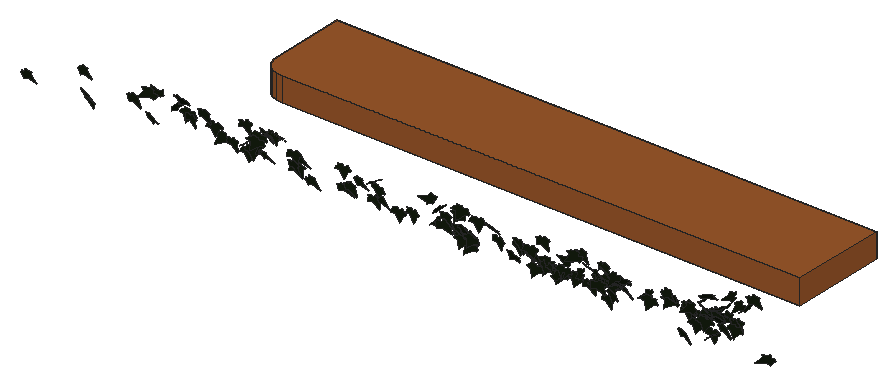
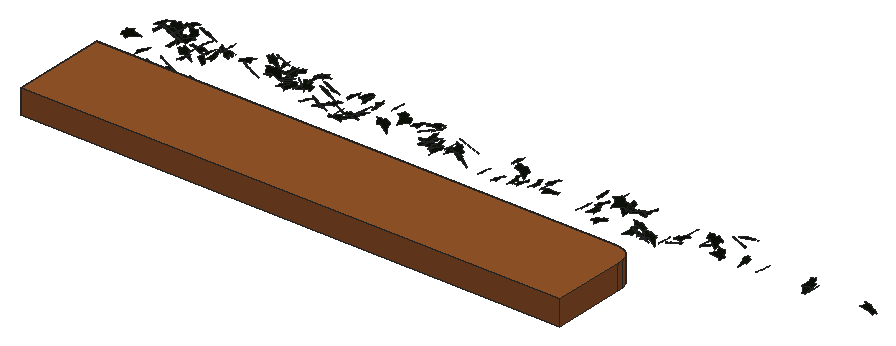
# SketchUp Ruby script. Lengths in millimetres.
U = 1.mm
M = Sketchup.active_model
def pt(a) = Geom::Point3d.new(a.map { |v| v * U })
def face(e, loops, mat)
  f = e.add_face(loops[0].map { |a| pt(a) })
  loops[1..].each { |l| e.add_face(l.map { |a| pt(a) }).erase! }
  f.material = f.back_material = mat if mat
  f
end
# faces: each face lists its corners as indices into pts; further lists are holes
def faces(e, pts, list, mat = nil) = list.each { |f| face(e, (f[0].is_a?(Array) ? f : [f]).map { |l| l.map { |i| pts[i] } }, mat) }
# xy, xz, yz: faces in a plane at the given z, y or x. An outline is a flat list of corners, or four numbers for a rectangle; further outlines are holes
def ring(l) = l.size == 4 ? [[l[0], l[1]], [l[2], l[1]], [l[2], l[3]], [l[0], l[3]]] : l.each_slice(2).to_a
def flat(e, list, mat, &to3) = list.each { |f| face(e, (f[0].is_a?(Array) ? f : [f]).map { |l| ring(l).map { |u, v| to3.(u, v) } }, mat) }
def xy(e, z, list, mat = nil) = flat(e, list, mat) { |x, y| [x, y, z] }
def xz(e, y, list, mat = nil) = flat(e, list, mat) { |x, z| [x, y, z] }
def yz(e, x, list, mat = nil) = flat(e, list, mat) { |y, z| [x, y, z] }
def lines(e, pts, list) = list.each { |a, b| e.add_line(pt(pts[a]), pt(pts[b])) }
# prism: a flat outline (further loops are holes) pulled along v
def prism(e, loops, v, mat = nil)
  f = face(e, loops, mat); d = Geom::Vector3d.new(v.map { |x| x * U })
  f.pushpull(f.normal.samedirection?(d) ? d.length : -d.length)
end
def box(e, o, s, mat = nil) = prism(e, [[o, [o[0] + s[0], o[1], o[2]], [o[0] + s[0], o[1] + s[1], o[2]], [o[0], o[1] + s[1], o[2]]]], [0, 0, s[2]], mat)
def at(x, y, z, deg = 0) = Geom::Transformation.translation(pt([x, y, z])) * Geom::Transformation.rotation(ORIGIN, Z_AXIS, deg.degrees)
def axes(o, x, y, z) = Geom::Transformation.new([*x, 0, *y, 0, *z, 0, *pt(o).to_a, 1])
def part(name) = M.definitions.add(name)
# library, detail: a bought-in or finely detailed component or shape, given as its bounding box
def library(name, o, s) = part(name).tap { |d| box(d.entities, o, s) }
def detail(e, o, s) = box(e.add_group.entities, o, s)
def put(e, d, t, mat = nil) = e.add_instance(d, t).tap { |i| i.material = mat if mat }
def group(e, t, mat = nil) = e.add_group.tap { |g| g.transformation = t; g.material = mat if mat }.entities
root = M.entities
M.materials.add("Emissive").color = [255, 185, 108]
M.materials.add("[Wood Cherry Original]").color = [152, 86, 42]
M.materials.add("efeu1").color = [18, 25, 13]
c1 = part("ivyleaf_9")
p = [[39.1,54.8,31.7],[34.5,51.8,30.2],[-5.3,25.2,17.3],[-17.9,28.3,20.9],[-21.6,21.7,17],[-20.2,4.3,5.3],
  [-22.9,-0.3,2.5],[-17.1,-4,-0.6],[-2,-2.1,-1.2],[-0.7,-15.4,-10.1],[16.6,-22.3,-16.7],[21.1,-15.1,-12.5],
  [32.7,-10.7,-11],[46.1,-1.8,-6.6],[30.8,11.2,3.8]]
faces(c1.entities,p,[[0,1,2,3,4,5,6,7,8,9,10,11,12,13,14]],"efeu1")
put(root,c1,axes([8074.5,526.7,5825.1],[-2.17662,-0.89017,-0.15094],[0.20307,0.10863,-1.44912],[1.70631,-1.14845,-0.02008]))
put(root,c1,axes([2613.1,371,5827.4],[0.23892,-1.21301,0.85578],[0.50011,-0.82712,-1.21092],[2.78069,0.25298,0.14425]))
put(root,c1,axes([6163.8,513.2,5830],[-0.62934,-1.41671,-0.06953],[0.03051,0.06765,-1.45479],[2.69936,-0.33106,0.00023]))
put(root,c1,axes([4921.2,550.8,5850.1],[-0.48361,-1.23805,-0.68713],[0.5351,0.64009,-1.25727],[2.64118,-0.35637,0.12891]))
put(root,c1,axes([10571.6,482.2,5821.8],[-0.21337,-0.04901,-1.49779],[-0.24319,-1.49619,0.05852],[-2.84173,0.13172,0.10745]))
put(root,c1,axes([5168,430.4,5854.4],[1.26122,-1.15667,-0.60639],[-0.06808,0.66366,-1.305],[2.48461,0.60532,0.27205]))
put(root,c1,axes([7115.8,397.2,5845.3],[-2.66405,-0.3276,-0.31618],[0.57453,0.09743,-1.43737],[0.64867,-1.43173,-0.02547]))
put(root,c1,axes([9847.7,543.6,5834.5],[-0.34368,-1.44406,-0.07033],[0.01652,0.06979,-1.45531],[2.75154,-0.18079,-0.00005]))
put(root,c1,axes([9623.6,355.2,5836.9],[1.52236,-1.2895,-0.02319],[-0.02465,0.01926,-1.51744],[2.45444,0.8,-0.00086]))
put(root,c1,axes([9922.6,457.9,5853.9],[-0.55823,1.32512,-0.53209],[0.00313,-0.54288,-1.35291],[-2.71768,-0.27281,0.10774]))
put(root,c1,axes([4382.2,525,5839.3],[-0.82714,-1.39965,0.00399],[0.04642,-0.01175,-1.46533],[2.66342,-0.43447,0.02677]))
put(root,c1,axes([6959.6,472.3,5852.5],[-1.32426,-1.09577,0.67655],[-0.32073,-0.6849,-1.28261],[2.42986,-0.68759,0.19942]))
put(root,c1,axes([4525.8,533.9,5858.8],[1.99885,-0.95702,-0.27557],[0.05319,0.42865,-1.38215],[1.89465,0.99761,0.32952]))
put(root,c1,axes([8422.7,503.1,5866.6],[-0.20032,-1.44792,-0.35467],[0.41494,0.33678,-1.43958],[2.80664,-0.15313,0.18752]))
put(root,c1,axes([7991.5,519.2,5862.7],[-0.53308,-1.41745,0.3331],[0.07754,-0.3467,-1.44108],[2.77009,-0.26307,0.10444]))
put(root,c1,axes([7929.3,514.9,5863.4],[-1.43561,-1.20456,0.40338],[-0.27216,-0.38564,-1.41898],[2.40228,-0.76354,0.0803]))
put(root,c1,axes([6307.3,534.6,5861.2],[-0.30689,-1.42825,0.19482],[-0.00237,-0.1959,-1.43718],[2.74342,-0.15994,0.02055]))
put(root,c1,axes([4417,538.3,5860.9],[-0.70879,-1.41411,0.01021],[0.03058,-0.01479,-1.4622],[2.69123,-0.37227,0.0193]))
put(root,c1,axes([5883.1,495.2,5879.9],[-0.07528,-1.37857,-0.49737],[0.17964,0.49412,-1.37707],[2.78344,-0.06918,0.07542]))
put(root,c1,axes([6883.1,502.8,5885.4],[0.2677,-1.15782,-0.88511],[-0.14456,0.88219,-1.16607],[2.76992,0.15794,0.02468]))
put(root,c1,axes([8271.9,523.6,5867.7],[-1.60859,-1.20404,0.15445],[0.05883,-0.20949,-1.46393],[2.30957,-0.83327,0.14486]))
put(root,c1,axes([8722,394,5865.9],[0.2362,-1.49888,0.06118],[0.01867,-0.06058,-1.504],[2.85498,0.1244,0.00477]))
put(root,c1,axes([7871.1,416.1,5870.6],[-1.47445,-1.21466,0.2883],[-0.02362,-0.33179,-1.43125],[2.37585,-0.75712,0.16469]))
put(root,c1,axes([7021.3,395.5,5873.9],[-1.28203,-1.19407,0.51458],[-0.15548,-0.53952,-1.35889],[2.4697,-0.65381,0.18157]))
put(root,c1,axes([9462.2,931.6,5866.9],[-0.51812,1.43082,-0.02284],[0.00789,-0.02246,-1.45649],[-2.72347,-0.27227,0.00013]))
put(root,c1,axes([8039.8,520.9,5871.8],[0.22661,-1.47073,0.13778],[-0.05792,-0.14064,-1.47496],[2.81075,0.11568,-0.0415]))
put(root,c1,axes([4099.7,526.8,5877.1],[-2.19562,-0.7999,0.43441],[-0.20382,-0.57717,-1.34716],[1.72035,-1.08926,0.39482]))
put(root,c1,axes([4496.7,550.6,5873.1],[-1.75881,1.11126,0.13863],[-0.41166,-0.00076,-1.43574],[-2.09121,-0.93447,0.16603]))
put(root,c1,axes([7050.9,474.1,5872.4],[-1.72475,-1.171,0.03617],[-0.0141,-0.04,-1.48059],[2.22966,-0.90608,0.01862]))
put(root,c1,axes([4176.2,525.2,5876.1],[0.50051,-1.4373,-0.12505],[-0.02862,0.12437,-1.46114],[2.74565,0.26331,0.00756]))
put(root,c1,axes([5544.9,482,5895.5],[-0.4571,-0.98003,-1.02974],[1.52498,0.7693,-0.91904],[2.23476,-0.72541,0.41653]))
put(root,c1,axes([9716.5,887,5870.4],[0.60839,0.8956,1.13524],[0.51702,1.10475,-0.94804],[-2.703,0.4129,0.07418]))
put(root,c1,axes([8131,418.2,5854.4],[-2.2074,0.66073,-0.71144],[-1.17316,0.35523,1.33483],[1.4277,1.31346,-0.00312]))
put(root,c1,axes([3324.1,363,5901.2],[2.09552,-0.55116,-0.78981],[-0.96665,0.68695,-1.18744],[1.55738,1.16799,0.32569]))
put(root,c1,axes([7589,423,5899.1],[1.51499,0.20162,-1.26609],[-2.40335,-0.13395,-0.81528],[-0.42119,1.48953,0.09806]))
put(root,c1,axes([1891.2,333.9,5872.9],[-0.0723,-0.29316,-1.43905],[2.73532,0.2886,-0.09674],[0.57478,-1.41032,0.27934]))
put(root,c1,axes([5937.2,506.4,5895.8],[1.53147,-1.19179,-0.37751],[-0.30259,0.34775,-1.43672],[2.35996,0.81799,0.06077]))
put(root,c1,axes([9436.4,936.6,5886.9],[2.0993,0.70408,0.61716],[0.93658,0.37536,-1.30776],[-1.51595,1.20693,0.04669]))
put(root,c1,axes([6643,495.3,5899.6],[-1.47757,1.20987,-0.23901],[0.26921,-0.1932,-1.43746],[-2.33163,-0.78901,-0.01451]))
put(root,c1,axes([4335.5,547.4,5894],[-0.22042,1.44759,-0.09005],[0.03728,-0.08877,-1.45216],[-2.76013,-0.1168,-0.01242]))
put(root,c1,axes([6715,460.8,5920.9],[-0.17939,-1.02389,-1.07244],[0.6259,1.0334,-1.01552],[2.75163,-0.30181,0.16108]))
put(root,c1,axes([9849.8,968.4,5918.2],[-2.41772,0.37642,-0.5762],[0.89977,-0.4018,-1.30481],[-0.95196,-1.33579,0.23011]))
put(root,c1,axes([7923.5,526.7,5903.8],[-2.61277,-0.5316,0.11045],[-0.14737,-0.10556,-1.47049],[1.02279,-1.37322,0.07028]))
put(root,c1,axes([6997.7,484.7,5907.7],[-0.22258,-1.44613,0.25942],[-0.06853,-0.25734,-1.45078],[2.79538,-0.12146,-0.01491]))
put(root,c1,axes([8317.5,520.1,5912],[-2.17254,0.93752,-0.15008],[0.11638,-0.16161,-1.47468],[-1.80326,-1.13994,0.08563]))
put(root,c1,axes([9614,550.8,5895.2],[0.22234,-0.05899,-1.44158],[2.60088,-0.45931,0.12954],[-0.88062,-1.37144,0.01862]))
put(root,c1,axes([2565.1,339.6,5909.3],[2.04119,-1.04548,-0.03075],[-0.04549,0.01953,-1.49776],[1.9901,1.07276,-0.0027]))
put(root,c1,axes([9941.5,963.7,5926.8],[-1.51695,1.11002,-0.49201],[0.38174,-0.46009,-1.36294],[-2.27907,-0.8159,0.09919]))
put(root,c1,axes([5608,472.8,5925.1],[0.49792,-1.37055,-0.38286],[0.00397,0.38965,-1.39341],[2.70829,0.2514,0.07243]))
put(root,c1,axes([9754,454.5,5932.1],[-2.22925,-0.62663,-0.58884],[1.05467,0.21076,-1.3266],[1.25137,-1.29395,0.06909]))
put(root,c1,axes([6870.3,477.7,5919.7],[1.11639,-1.39175,0.06191],[0.04657,-0.05687,-1.51032],[2.651,0.5871,0.00046]))
put(root,c1,axes([8144.7,482.1,5920.5],[-1.36467,-1.27837,0.00389],[0.05068,-0.01939,-1.46537],[2.43248,-0.71679,0.03271]))
put(root,c1,axes([7141.3,383.9,5930.5],[-1.51061,-1.13052,0.5055],[-0.15923,-0.55009,-1.36162],[2.35151,-0.76349,0.23253]))
put(root,c1,axes([9970.5,528,5930.8],[1.20104,-1.31121,-0.15388],[-0.06338,0.15469,-1.4547],[2.51182,0.63086,0.03687]))
put(root,c1,axes([4482.1,512.6,5935.1],[-0.34853,1.39929,0.38168],[-0.66756,0.33057,-1.38019],[-2.67849,-0.26446,0.29432]))
put(root,c1,axes([4942.1,551.1,5945.4],[1.7208,-1.0969,-0.2869],[0.0833,0.40045,-1.3931],[2.15625,0.85992,0.28278]))
put(root,c1,axes([8696.9,515.1,5934.2],[-1.0833,-1.36042,-0.02757],[0.02667,0.02402,-1.47469],[2.58954,-0.56936,0.00365]))
put(root,c1,axes([8563.2,481.2,5935.3],[-1.43694,-0.51266,1.16043],[-1.16352,-1.03622,-0.85555],[2.11562,-0.91809,0.31765]))
put(root,c1,axes([3031.6,481.9,5958.3],[0.83833,-1.33393,-0.39082],[0.08307,0.42305,-1.39473],[2.64416,0.40963,0.16773]))
put(root,c1,axes([6954.7,446.8,5956.1],[1.72062,-1.16045,-0.26707],[-0.15522,0.27419,-1.46747],[2.26098,0.90194,0.1025]))
put(root,c1,axes([5649,542.7,5969.1],[1.50154,-1.17861,-0.33272],[0.008,0.39839,-1.40126],[2.33078,0.75792,0.21916]))
put(root,c1,axes([8629.5,473.5,5969.5],[2.63079,0.44114,-0.2309],[-0.38678,-0.12215,-1.44998],[-0.86511,1.39612,-0.0539]))
put(root,c1,axes([3982,515.9,5974.4],[-0.98985,-1.35354,-0.31276],[0.14012,0.30663,-1.44946],[2.64021,-0.52373,-0.04033]))
put(root,c1,axes([7746.8,467.5,5982.5],[0.91678,-1.36019,-0.41762],[0.15716,0.46688,-1.4254],[2.70341,0.43413,0.22449]))
put(root,c1,axes([9712,547.4,5963.8],[0.16735,-1.44975,0.03493],[0.00077,-0.03497,-1.45241],[2.75996,0.08791,-0.00171]))
put(root,c1,axes([8856.6,311.8,5973.8],[-0.31839,-1.1428,0.94464],[-0.08234,-0.94647,-1.15267],[2.82063,-0.15663,0.07298]))
put(root,c1,axes([6708,513.1,5976.4],[0.53261,-1.4357,-0.1573],[0.07996,0.16825,-1.4609],[2.74762,0.27341,0.07301]))
put(root,c1,axes([2392.4,546.3,5997],[1.0312,-1.18623,-0.64307],[-0.23783,0.64589,-1.29672],[2.55701,0.53846,0.13873]))
put(root,c1,axes([9562,528.4,5979.1],[-0.22617,-1.46967,-0.03001],[-0.08508,0.03371,-1.4737],[2.79636,-0.11784,-0.04726]))
put(root,c1,axes([9130.9,512.3,5978.2],[-2.13533,0.97288,0.0186],[-0.02858,0.01107,-1.48503],[-1.85171,-1.12207,0.00147]))
put(root,c1,axes([8682.7,509.2,5987.9],[-1.85652,-1.0603,0.3972],[0.0186,-0.53214,-1.39653],[2.15483,-0.90892,0.35426]))
put(root,c1,axes([3722.3,483.8,5983.3],[0.46935,-1.45658,0.09217],[0.00557,-0.09299,-1.47725],[2.7777,0.2463,-0.01261]))
put(root,c1,axes([8847.7,461.3,5986.2],[1.66454,-1.19951,0.10159],[0.10933,-0.08385,-1.48451],[2.28848,0.87648,-0.00298]))
put(root,c1,axes([8502.3,495.6,6002.1],[-1.21259,0.12987,-1.35187],[2.24754,-0.68446,-0.62232],[-1.27647,-1.32854,0.18847]))
put(root,c1,axes([9204.3,437.1,5988.4],[-1.61526,-1.22771,0.1124],[-0.1003,-0.1002,-1.49245],[2.34421,-0.85023,0.01359]))
g1 = group(root,at(3881.8,1531.6,5905.3),"[Wood Cherry Original]")
xy(g1,0,[[[6377.5,-209.6,265.9,-209.5,184.6,-202.2,118.2,-180,66.5,-143.1,29.5,-91.4,7.4,-24.9,0,56.3,0,914.4,6377.5,914.4],[4138.7,109.7,4197.4,117.4,4252.2,140.1,4299.2,176.2,4335.3,223.2,4357.9,278,4365.7,336.7,4357.9,395.5,4335.3,450.2,4299.2,497.2,4252.2,533.3,4197.4,556,4138.7,563.7,4079.9,556,4025.1,533.3,3978.1,497.2,3942.1,450.2,3919.4,395.5,3911.6,336.7,3919.4,278,3942.1,223.2,3978.1,176.2,4025.1,140.1,4079.9,117.4],[2346.9,109.7,2405.7,117.4,2460.4,140.1,2507.4,176.2,2543.5,223.2,2566.2,278,2573.9,336.7,2566.2,395.5,2543.5,450.2,2507.4,497.2,2460.4,533.3,2405.7,556,2346.9,563.7,2288.1,556,2233.4,533.3,2186.4,497.2,2150.3,450.2,2127.6,395.5,2119.9,336.7,2127.6,278,2150.3,223.2,2186.4,176.2,2233.4,140.1,2288.1,117.4],[555.1,109.7,613.9,117.4,668.6,140.1,715.7,176.2,751.7,223.2,774.4,278,782.1,336.7,774.4,395.5,751.7,450.2,715.7,497.2,668.6,533.3,613.9,556,555.1,563.7,496.4,556,441.6,533.3,394.6,497.2,358.5,450.2,335.9,395.5,328.1,336.7,335.9,278,358.5,223.2,394.6,176.2,441.6,140.1,496.4,117.4],[5930.4,109.7,5989.2,117.4,6043.9,140.1,6090.9,176.2,6127,223.2,6149.7,278,6157.4,336.7,6149.7,395.5,6127,450.2,6090.9,497.2,6043.9,533.3,5989.2,556,5930.4,563.7,5871.7,556,5816.9,533.3,5769.9,497.2,5733.8,450.2,5711.1,395.5,5703.4,336.7,5711.1,278,5733.8,223.2,5769.9,176.2,5816.9,140.1,5871.7,117.4]],[[555.1,109.7,496.4,117.4,441.6,140.1,394.6,176.2,358.5,223.2,335.9,278,328.1,336.7,335.9,395.5,358.5,450.2,394.6,497.2,441.6,533.3,496.4,556,555.1,563.7,613.9,556,668.6,533.3,715.7,497.2,751.7,450.2,774.4,395.5,782.1,336.7,774.4,278,751.7,223.2,715.7,176.2,668.6,140.1,613.9,117.4],[555.1,166.8,599.1,172.6,640.1,189.6,675.2,216.6,702.2,251.8,719.2,292.7,725,336.7,719.2,380.7,702.2,421.6,675.2,456.8,640.1,483.8,599.1,500.8,555.1,506.6,511.2,500.8,470.2,483.8,435,456.8,408,421.6,391.1,380.7,385.3,336.7,391.1,292.7,408,251.8,435,216.6,470.2,189.6,511.2,172.6]],[[2346.9,109.7,2288.1,117.4,2233.4,140.1,2186.4,176.2,2150.3,223.2,2127.6,278,2119.9,336.7,2127.6,395.5,2150.3,450.2,2186.4,497.2,2233.4,533.3,2288.1,556,2346.9,563.7,2405.7,556,2460.4,533.3,2507.4,497.2,2543.5,450.2,2566.2,395.5,2573.9,336.7,2566.2,278,2543.5,223.2,2507.4,176.2,2460.4,140.1,2405.7,117.4],[2346.9,166.8,2390.9,172.6,2431.8,189.6,2467,216.6,2494,251.8,2511,292.7,2516.8,336.7,2511,380.7,2494,421.6,2467,456.8,2431.8,483.8,2390.9,500.8,2346.9,506.6,2302.9,500.8,2262,483.8,2226.8,456.8,2199.8,421.6,2182.8,380.7,2177,336.7,2182.8,292.7,2199.8,251.8,2226.8,216.6,2262,189.6,2302.9,172.6]],[[4138.7,109.7,4079.9,117.4,4025.1,140.1,3978.1,176.2,3942.1,223.2,3919.4,278,3911.6,336.7,3919.4,395.5,3942.1,450.2,3978.1,497.2,4025.1,533.3,4079.9,556,4138.7,563.7,4197.4,556,4252.2,533.3,4299.2,497.2,4335.3,450.2,4357.9,395.5,4365.7,336.7,4357.9,278,4335.3,223.2,4299.2,176.2,4252.2,140.1,4197.4,117.4],[4138.7,166.8,4182.6,172.6,4223.6,189.6,4258.8,216.6,4285.8,251.8,4302.7,292.7,4308.5,336.7,4302.7,380.7,4285.8,421.6,4258.8,456.8,4223.6,483.8,4182.6,500.8,4138.7,506.6,4094.7,500.8,4053.7,483.8,4018.5,456.8,3991.5,421.6,3974.6,380.7,3968.8,336.7,3974.6,292.7,3991.5,251.8,4018.5,216.6,4053.7,189.6,4094.7,172.6]],[[5930.4,109.7,5871.7,117.4,5816.9,140.1,5769.9,176.2,5733.8,223.2,5711.1,278,5703.4,336.7,5711.1,395.5,5733.8,450.2,5769.9,497.2,5816.9,533.3,5871.7,556,5930.4,563.7,5989.2,556,6043.9,533.3,6090.9,497.2,6127,450.2,6149.7,395.5,6157.4,336.7,6149.7,278,6127,223.2,6090.9,176.2,6043.9,140.1,5989.2,117.4],[5930.4,166.8,5974.4,172.6,6015.3,189.6,6050.5,216.6,6077.5,251.8,6094.5,292.7,6100.3,336.7,6094.5,380.7,6077.5,421.6,6050.5,456.8,6015.3,483.8,5974.4,500.8,5930.4,506.6,5886.4,500.8,5845.5,483.8,5810.3,456.8,5783.3,421.6,5766.3,380.7,5760.5,336.7,5766.3,292.7,5783.3,251.8,5810.3,216.6,5845.5,189.6,5886.4,172.6]]])
xy(g1,100,[[555.1,166.8,511.2,172.6,470.2,189.6,435,216.6,408,251.8,391.1,292.7,385.3,336.7,391.1,380.7,408,421.6,435,456.8,470.2,483.8,511.2,500.8,555.1,506.6,599.1,500.8,640.1,483.8,675.2,456.8,702.2,421.6,719.2,380.7,725,336.7,719.2,292.7,702.2,251.8,675.2,216.6,640.1,189.6,599.1,172.6]],"Emissive")
xy(g1,138.1,[[2346.9,166.8,2302.9,172.6,2262,189.6,2226.8,216.6,2199.8,251.8,2182.8,292.7,2177,336.7,2182.8,380.7,2199.8,421.6,2226.8,456.8,2262,483.8,2302.9,500.8,2346.9,506.6,2390.9,500.8,2431.8,483.8,2467,456.8,2494,421.6,2511,380.7,2516.8,336.7,2511,292.7,2494,251.8,2467,216.6,2431.8,189.6,2390.9,172.6],[4138.7,166.8,4094.7,172.6,4053.7,189.6,4018.5,216.6,3991.5,251.8,3974.6,292.7,3968.8,336.7,3974.6,380.7,3991.5,421.6,4018.5,456.8,4053.7,483.8,4094.7,500.8,4138.7,506.6,4182.6,500.8,4223.6,483.8,4258.8,456.8,4285.8,421.6,4302.7,380.7,4308.5,336.7,4302.7,292.7,4285.8,251.8,4258.8,216.6,4223.6,189.6,4182.6,172.6],[5930.4,166.8,5886.4,172.6,5845.5,189.6,5810.3,216.6,5783.3,251.8,5766.3,292.7,5760.5,336.7,5766.3,380.7,5783.3,421.6,5810.3,456.8,5845.5,483.8,5886.4,500.8,5930.4,506.6,5974.4,500.8,6015.3,483.8,6050.5,456.8,6077.5,421.6,6094.5,380.7,6100.3,336.7,6094.5,292.7,6077.5,251.8,6050.5,216.6,6015.3,189.6,5974.4,172.6]],"Emissive")
xy(g1,290.5,[[6377.5,-209.6,6377.5,914.4,0,914.4,0,56.3,7.4,-24.9,29.5,-91.4,66.5,-143.1,118.2,-180,184.6,-202.2,265.9,-209.5]])
xz(g1,914.4,[[0,0,6377.5,290.5]])
yz(g1,0,[[56.3,0,914.4,290.5]])
yz(g1,6377.5,[[-209.6,0,914.4,290.5]])
p = [[265.9,-209.5,0],[6377.5,-209.6,0],[6377.5,-209.6,290.5],[265.9,-209.5,290.5],[184.6,-202.2,290.5],[184.6,-202.2,0],
  [118.2,-180,290.5],[118.2,-180,0],[66.5,-143.1,290.5],[66.5,-143.1,0],[29.5,-91.4,290.5],[29.5,-91.4,0],
  [7.4,-24.9,290.5],[7.4,-24.9,0],[0,56.3,290.5],[0,56.3,0],[555.1,166.8,0],[511.2,172.6,0],
  [511.2,172.6,100],[555.1,166.8,100],[599.1,172.6,0],[599.1,172.6,100],[2346.9,166.8,0],[2302.9,172.6,0],
  [2302.9,172.6,138.1],[2346.9,166.8,138.1],[2390.9,172.6,0],[2390.9,172.6,138.1],[4138.7,166.8,0],[4094.7,172.6,0],
  [4094.7,172.6,138.1],[4138.7,166.8,138.1],[4182.6,172.6,0],[4182.6,172.6,138.1],[5930.4,166.8,0],[5886.4,172.6,0],
  [5886.4,172.6,138.1],[5930.4,166.8,138.1],[5974.4,172.6,0],[5974.4,172.6,138.1],[470.2,189.6,0],[470.2,189.6,100],
  [640.1,189.6,0],[640.1,189.6,100],[2262,189.6,0],[2262,189.6,138.1],[2431.8,189.6,0],[2431.8,189.6,138.1],
  [4053.7,189.6,0],[4053.7,189.6,138.1],[4223.6,189.6,0],[4223.6,189.6,138.1],[5845.5,189.6,0],[5845.5,189.6,138.1],
  [6015.3,189.6,0],[6015.3,189.6,138.1],[435,216.6,0],[435,216.6,100],[675.2,216.6,0],[675.2,216.6,100],
  [2226.8,216.6,0],[2226.8,216.6,138.1],[2467,216.6,0],[2467,216.6,138.1],[4018.5,216.6,0],[4018.5,216.6,138.1],
  [4258.8,216.6,0],[4258.8,216.6,138.1],[5810.3,216.6,0],[5810.3,216.6,138.1],[6050.5,216.6,0],[6050.5,216.6,138.1],
  [408,251.8,0],[408,251.8,100],[702.2,251.8,0],[702.2,251.8,100],[2199.8,251.8,0],[2199.8,251.8,138.1],
  [2494,251.8,0],[2494,251.8,138.1],[3991.5,251.8,0],[3991.5,251.8,138.1],[4285.8,251.8,0],[4285.8,251.8,138.1],
  [5783.3,251.8,0],[5783.3,251.8,138.1],[6077.5,251.8,0],[6077.5,251.8,138.1],[391.1,292.7,0],[391.1,292.7,100],
  [719.2,292.7,0],[719.2,292.7,100],[2182.8,292.7,0],[2182.8,292.7,138.1],[2511,292.7,0],[2511,292.7,138.1],
  [3974.6,292.7,0],[3974.6,292.7,138.1],[4302.7,292.7,0],[4302.7,292.7,138.1],[5766.3,292.7,0],[5766.3,292.7,138.1],
  [6094.5,292.7,0],[6094.5,292.7,138.1],[385.3,336.7,0],[385.3,336.7,100],[725,336.7,0],[725,336.7,100],
  [2177,336.7,0],[2177,336.7,138.1],[2516.8,336.7,0],[2516.8,336.7,138.1],[3968.8,336.7,0],[3968.8,336.7,138.1],
  [4308.5,336.7,0],[4308.5,336.7,138.1],[5760.5,336.7,0],[5760.5,336.7,138.1],[6100.3,336.7,0],[6100.3,336.7,138.1],
  [391.1,380.7,0],[391.1,380.7,100],[719.2,380.7,0],[719.2,380.7,100],[2182.8,380.7,0],[2182.8,380.7,138.1],
  [2511,380.7,0],[2511,380.7,138.1],[3974.6,380.7,0],[3974.6,380.7,138.1],[4302.7,380.7,0],[4302.7,380.7,138.1],
  [5766.3,380.7,0],[5766.3,380.7,138.1],[6094.5,380.7,0],[6094.5,380.7,138.1],[408,421.6,0],[408,421.6,100],
  [702.2,421.6,0],[702.2,421.6,100],[2199.8,421.6,0],[2199.8,421.6,138.1],[2494,421.6,0],[2494,421.6,138.1],
  [3991.5,421.6,0],[3991.5,421.6,138.1],[4285.8,421.6,0],[4285.8,421.6,138.1],[5783.3,421.6,0],[5783.3,421.6,138.1],
  [6077.5,421.6,0],[6077.5,421.6,138.1],[435,456.8,0],[435,456.8,100],[675.2,456.8,0],[675.2,456.8,100],
  [2226.8,456.8,0],[2226.8,456.8,138.1],[2467,456.8,0],[2467,456.8,138.1],[4018.5,456.8,0],[4018.5,456.8,138.1],
  [4258.8,456.8,0],[4258.8,456.8,138.1],[5810.3,456.8,0],[5810.3,456.8,138.1],[6050.5,456.8,0],[6050.5,456.8,138.1],
  [470.2,483.8,0],[470.2,483.8,100],[640.1,483.8,0],[640.1,483.8,100],[2262,483.8,0],[2262,483.8,138.1],
  [2431.8,483.8,0],[2431.8,483.8,138.1],[4053.7,483.8,0],[4053.7,483.8,138.1],[4223.6,483.8,0],[4223.6,483.8,138.1],
  [5845.5,483.8,0],[5845.5,483.8,138.1],[6015.3,483.8,0],[6015.3,483.8,138.1],[511.2,500.8,0],[511.2,500.8,100],
  [599.1,500.8,0],[599.1,500.8,100],[2302.9,500.8,0],[2302.9,500.8,138.1],[2390.9,500.8,0],[2390.9,500.8,138.1],
  [4094.7,500.8,0],[4094.7,500.8,138.1],[4182.6,500.8,0],[4182.6,500.8,138.1],[5886.4,500.8,0],[5886.4,500.8,138.1],
  [5974.4,500.8,0],[5974.4,500.8,138.1],[555.1,506.6,0],[555.1,506.6,100],[2346.9,506.6,0],[2346.9,506.6,138.1],
  [4138.7,506.6,0],[4138.7,506.6,138.1],[5930.4,506.6,0],[5930.4,506.6,138.1]]
faces(g1,p,[[0,1,2,3],[0,3,4,5],[5,4,6,7],[7,6,8,9],[9,8,10,11],[11,10,12,13],[13,12,14,15]])
faces(g1,p,[[16,17,18,19],[20,16,19,21],[22,23,24,25],[26,22,25,27],[28,29,30,31],[32,28,31,33],[34,35,36,37],[38,34,37,39],
  [17,40,41,18],[42,20,21,43],[23,44,45,24],[46,26,27,47],[29,48,49,30],[50,32,33,51],[35,52,53,36],[54,38,39,55],
  [40,56,57,41],[58,42,43,59],[44,60,61,45],[62,46,47,63],[48,64,65,49],[66,50,51,67],[52,68,69,53],[70,54,55,71],
  [56,72,73,57],[74,58,59,75],[60,76,77,61],[78,62,63,79],[64,80,81,65],[82,66,67,83],[68,84,85,69],[86,70,71,87],
  [72,88,89,73],[90,74,75,91],[76,92,93,77],[94,78,79,95],[80,96,97,81],[98,82,83,99],[84,100,101,85],[102,86,87,103],
  [88,104,105,89],[106,90,91,107],[92,108,109,93],[110,94,95,111],[96,112,113,97],[114,98,99,115],[100,116,117,101],[118,102,103,119],
  [104,120,121,105],[122,106,107,123],[108,124,125,109],[126,110,111,127],[112,128,129,113],[130,114,115,131],[116,132,133,117],[134,118,119,135],
  [120,136,137,121],[138,122,123,139],[124,140,141,125],[142,126,127,143],[128,144,145,129],[146,130,131,147],[132,148,149,133],[150,134,135,151],
  [136,152,153,137],[154,138,139,155],[140,156,157,141],[158,142,143,159],[144,160,161,145],[162,146,147,163],[148,164,165,149],[166,150,151,167],
  [152,168,169,153],[170,154,155,171],[156,172,173,157],[174,158,159,175],[160,176,177,161],[178,162,163,179],[164,180,181,165],[182,166,167,183],
  [168,184,185,169],[186,170,171,187],[172,188,189,173],[190,174,175,191],[176,192,193,177],[194,178,179,195],[180,196,197,181],[198,182,183,199],
  [184,200,201,185],[200,186,187,201],[188,202,203,189],[202,190,191,203],[192,204,205,193],[204,194,195,205],[196,206,207,197],[206,198,199,207]],"Emissive")
put(root,c1,axes([3687.5,519.5,5994.7],[-1.53484,-1.2066,0.28178],[0.18297,-0.39612,-1.42109],[2.35108,-0.75687,0.29455]))
put(root,c1,axes([4918.1,515.4,6005.1],[-0.32489,-1.38964,-0.42136],[0.07183,0.41987,-1.40002],[2.76273,-0.17433,-0.01315]))
put(root,c1,axes([5017.2,374.2,5993.8],[0.94899,-1.42704,0.04607],[-0.00466,-0.04966,-1.51153],[2.71734,0.49828,-0.01868]))
put(root,c1,axes([8653.7,331.7,6017],[-0.3096,-1.21915,-0.82843],[0.34664,0.81045,-1.22845],[2.78379,-0.2365,0.06083]))
put(root,c1,axes([3490.1,532.4,5966.9],[0.65104,0.23819,1.41732],[1.8864,1.01591,-0.40995],[-1.98072,1.04582,0.07542]))
put(root,c1,axes([6595,512.3,5979.7],[0.79,0.31737,1.37767],[1.53795,1.12489,-0.50261],[-2.2078,0.89716,0.14284]))
put(root,c1,axes([9911.4,490.5,6020.3],[2.48834,0.39742,-0.49683],[-0.96012,-0.04427,-1.363],[-0.7378,1.39797,0.09808]))
put(root,c1,axes([9783.9,933.1,6005.2],[-2.14533,0.90564,-0.04749],[0.0676,-0.03161,-1.44597],[-1.72467,-1.12778,0.0024]))
put(root,c1,axes([9812.2,538,6027.9],[-0.87308,-1.3511,-0.31739],[0.09828,0.31744,-1.42591],[2.63959,-0.45872,-0.05189]))
put(root,c1,axes([8825.8,491.3,6043.7],[1.20777,0.68927,-1.1747],[-1.65114,-0.79445,-0.93483],[-1.99822,1.07307,0.06244]))
put(root,c1,axes([4545.1,452.2,6026.5],[-2.4106,-0.76159,-0.10938],[0.22375,0.01663,-1.47722],[1.44713,-1.27121,0.0462]))
put(root,c1,axes([7643.8,417.5,6030],[0.21877,-1.31351,0.72253],[0.09556,-0.72087,-1.31848],[2.85153,0.12493,-0.01125]))
put(root,c1,axes([10137.5,534.1,6040],[0.07038,-1.38947,-0.4731],[0.03774,0.47368,-1.38962],[2.79327,0.02861,0.03069]))
put(root,c1,axes([5986.5,440.4,6034.2],[-0.63392,-1.27835,0.70772],[0.17771,-0.74302,-1.29815],[2.77524,-0.24442,0.24478]))
put(root,c1,axes([7784.2,400.5,6033.8],[0.38985,-1.42348,0.43015],[0.37371,-0.40452,-1.43216],[2.80537,0.2517,0.13101]))
put(root,c1,axes([9406.8,502.6,6029.8],[-2.52686,-0.69621,-0.03301],[0.20631,-0.13611,-1.48939],[1.31037,-1.3211,0.17085]))
put(root,c1,axes([9984.1,957.6,6049.7],[0.4548,-1.20813,-0.77838],[0.17179,0.80013,-1.21417],[2.72983,0.15092,0.20609]))
put(root,c1,axes([8383.8,503.3,6029.7],[2.5452,-0.63028,-0.0417],[0.11708,0.22713,-1.46016],[1.19645,1.31856,0.23159]))
put(root,c1,axes([10204.7,441,6033.4],[-1.06692,-1.35846,0.15579],[-0.16019,-0.13377,-1.46935],[2.59744,-0.56625,-0.02663]))
put(root,c1,axes([10038.2,537.3,6036.2],[-1.57612,0.82897,0.87674],[-1.19212,0.61351,-1.17173],[-1.96273,-1.03832,0.00764]))
put(root,c1,axes([9589,492.2,6059.3],[0.67854,-1.32377,-0.64662],[0.02315,0.6679,-1.36064],[2.8038,0.31485,0.16772]))
put(root,c1,axes([4525.7,510.9,6042.9],[-1.57162,-1.21139,0.28154],[0.05783,-0.3575,-1.44911],[2.36626,-0.79585,0.22241]))
put(root,c1,axes([5869.8,500.3,6039],[0.58015,1.43413,0.09242],[-0.0367,0.09855,-1.46564],[-2.73484,0.3029,0.03928]))
put(root,c1,axes([5488.1,540.7,6040.8],[-0.82618,-1.39095,-0.09361],[0.04693,0.09036,-1.45711],[2.65282,-0.43479,-0.00337]))
put(root,c1,axes([7626.7,449.4,6043.9],[0.44504,-1.47474,0.17437],[0.12665,-0.16594,-1.49265],[2.82345,0.2399,0.03947]))
put(root,c1,axes([8231.9,499.5,6046],[-1.41224,1.2255,0.32946],[-0.49113,0.22795,-1.42915],[-2.36473,-0.77923,0.10006]))
put(root,c1,axes([10130.3,512.1,6051.1],[1.09604,-1.33843,-0.24182],[-0.10309,0.23982,-1.45639],[2.58649,0.57673,0.04443]))
put(root,c1,axes([8239.4,431.8,6048.4],[-1.09426,0.85921,1.10587],[-1.29145,0.8748,-1.03248],[-2.3315,-0.88783,0.05288]))
put(root,c1,axes([7461.6,357.4,6055.8],[0.12677,-1.47178,0.27933],[0.08054,-0.27765,-1.473],[2.84996,0.07331,0.0292]))
put(root,c1,axes([7256.9,475.9,6069.8],[2.7624,-0.18507,-0.35803],[-0.63423,0.20156,-1.45515],[0.43142,1.48131,0.15328]))
put(root,c1,axes([8944.4,371.9,6071.6],[-0.94821,1.35036,-0.44056],[0.16543,-0.43701,-1.43779],[-2.69826,-0.50133,0.06667]))
put(root,c1,axes([3853.6,508.7,6065.4],[0.58679,-1.44235,-0.23538],[0.0221,0.24297,-1.47366],[2.7813,0.30237,0.06137]))
put(root,c1,axes([9404.4,506.3,6014.4],[0.25709,-0.33713,1.45485],[-1.00661,1.35531,0.36318],[-2.65802,-0.54587,0.00318]))
put(root,c1,axes([7811.1,388.7,6070.8],[-0.52021,-1.42749,-0.37313],[0.07148,0.37263,-1.45307],[2.80717,-0.27403,-0.03215]))
put(root,c1,axes([6904.9,487.6,6063.8],[-1.23964,-1.15831,0.65192],[-0.34483,-0.64184,-1.32142],[2.50605,-0.66129,0.14065]))
put(root,c1,axes([7106.7,505.7,6067],[-0.91918,-1.40463,-0.19776],[0.13173,0.18533,-1.48534],[2.69645,-0.48787,0.00515]))
put(root,c1,axes([9927.7,345.5,6066.5],[-1.40776,-1.26803,-0.14603],[0.16752,0.1177,-1.46791],[2.42348,-0.74471,0.01664]))
put(root,c1,axes([6549.8,518.6,6073.7],[-1.6391,0.97795,0.69685],[-1.14905,0.38864,-1.29158],[-1.97556,-1.03744,0.17305]))
put(root,c1,axes([4630.5,514.4,6081.9],[2.26608,0.73727,-0.42845],[-0.77378,-0.15599,-1.39828],[-1.42656,1.25576,0.07786]))
put(root,c1,axes([9902.6,513,6088.4],[0.85357,-1.274,-0.58163],[-0.03847,0.60478,-1.34028],[2.66513,0.41676,0.16693]))
put(root,c1,axes([9943.1,504,6078],[2.24339,-0.62645,0.68849],[1.36528,-0.09657,-1.31604],[1.12891,1.36166,0.22342]))
put(root,c1,axes([9331.9,485,6098.8],[1.09279,-1.11601,-0.85183],[-0.29872,0.86352,-1.23712],[2.65525,0.55645,0.2114]))
put(root,c1,axes([8582.3,484.1,6082],[1.92243,-1.08977,0.30654],[0.37864,-0.23354,-1.48585],[2.121,1.02943,-0.01258]))
put(root,c1,axes([4563,528,6087.8],[0.84737,-1.24767,0.64284],[0.71374,-0.54414,-1.31584],[2.5741,0.5616,0.15324]))
put(root,c1,axes([3586.5,509.8,6109.6],[2.1317,0.3491,-0.93058],[-1.79814,-0.0613,-1.16017],[-0.58725,1.45491,0.17441]))
put(root,c1,axes([9747,503.6,6078.9],[1.80832,-0.44085,-1.07984],[1.89897,-0.41406,1.04698],[-1.14957,-1.37746,0.03087]))
put(root,c1,axes([9725.8,402.6,6093.4],[-2.63102,0.54406,0.10607],[-0.15237,0.08604,-1.48476],[-1.04389,-1.38381,-0.05061]))
put(root,c1,axes([8816.9,398.5,6116.7],[-2.42171,0.03999,-0.77222],[1.3876,-0.43331,-1.22381],[-0.49025,-1.42397,0.35072]))
put(root,c1,axes([8586.5,499.3,6107.5],[0.53557,-1.45855,-0.25764],[-0.05161,0.25713,-1.48529],[2.81841,0.28187,0.02176]))
put(root,c1,axes([7852.9,519.2,6119.3],[0.14588,-1.36024,-0.57767],[-0.03956,0.5774,-1.36235],[2.81231,0.07868,0.0108]))
put(root,c1,axes([4335.6,518.2,6120.5],[0.11336,-1.41374,-0.45576],[-0.0143,0.45584,-1.41495],[2.82696,0.059,0.01112]))
put(root,c1,axes([4667.4,518.9,6107.9],[2.82276,0.07544,0.00278],[-0.02193,0.28027,-1.45835],[-0.14199,1.45645,0.28049]))
put(root,c1,axes([3373,435.5,6099.5],[0.14308,0.77287,1.25945],[-1.31659,1.13276,-0.65383],[-2.48512,-0.55563,0.41891]))
put(root,c1,axes([6928.6,493.4,6117.9],[-1.95482,-1.1019,0.00701],[-0.05308,0.01642,-1.50604],[2.0965,-1.02702,-0.0316]))
put(root,c1,axes([9955.6,505.2,6127.8],[0.09249,1.44248,-0.24604],[-0.14446,-0.24336,-1.44176],[-2.78123,0.06061,0.06671]))
put(root,c1,axes([8301.3,513.6,6142.3],[0.49479,-1.28733,-0.70574],[-0.09278,0.70875,-1.31079],[2.79253,0.25164,0.08149]))
put(root,c1,axes([4694.1,500,6129.5],[0.10158,-1.43775,0.38232],[-0.0074,-0.3827,-1.43863],[2.8314,0.05058,-0.01747]))
put(root,c1,axes([8314.1,457.7,6129.8],[-1.90353,-0.83735,0.69377],[-1.04514,-0.42464,-1.3042],[1.78629,-1.14077,-0.02376]))
put(root,c1,axes([3346.5,389.6,6137.1],[-2.49641,-0.42145,0.57101],[-0.77395,-0.53709,-1.33056],[1.10698,-1.32595,0.35746]))
